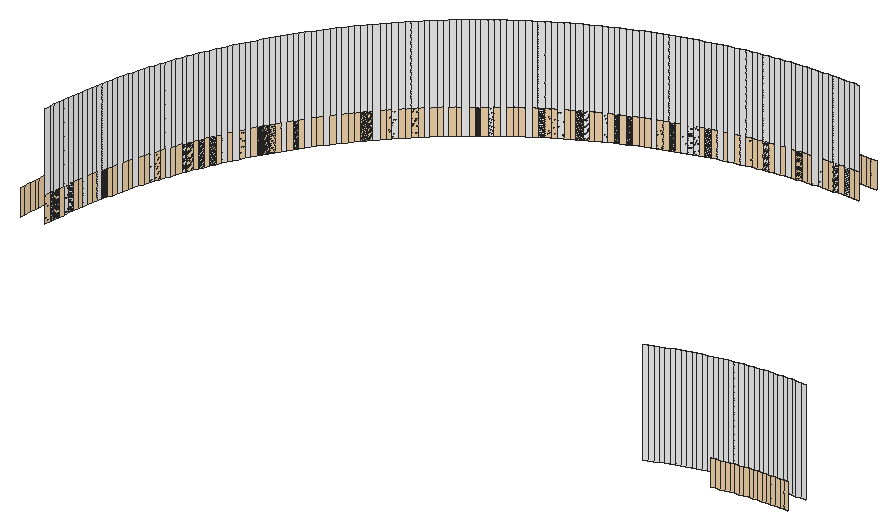
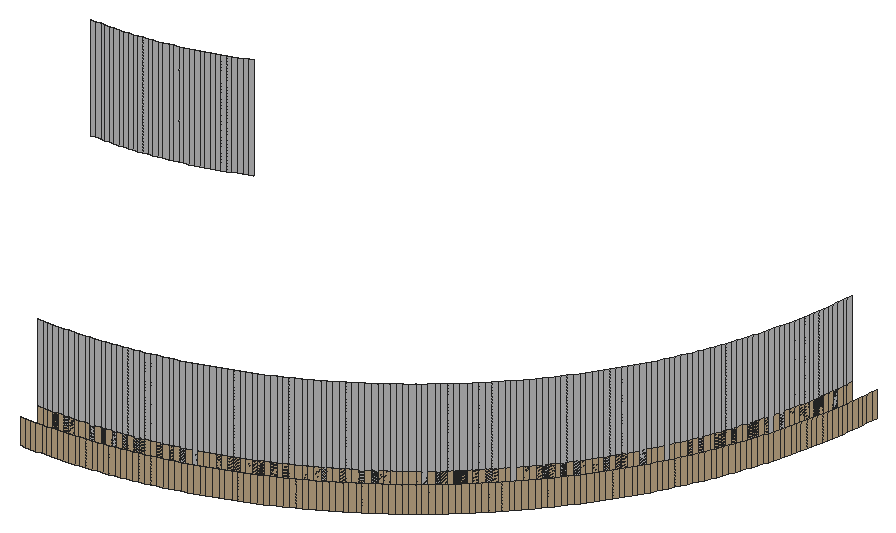
# SketchUp Ruby script. Lengths in inches.
U = 1.inch
M = Sketchup.active_model
def pt(a) = Geom::Point3d.new(a.map { |v| v * U })
def face(e, loops, mat)
  f = e.add_face(loops[0].map { |a| pt(a) })
  loops[1..].each { |l| e.add_face(l.map { |a| pt(a) }).erase! }
  f.material = f.back_material = mat if mat
  f
end
# faces: each face lists its corners as indices into pts; further lists are holes
def faces(e, pts, list, mat = nil) = list.each { |f| face(e, (f[0].is_a?(Array) ? f : [f]).map { |l| l.map { |i| pts[i] } }, mat) }
# xy, xz, yz: faces in a plane at the given z, y or x. An outline is a flat list of corners, or four numbers for a rectangle; further outlines are holes
def ring(l) = l.size == 4 ? [[l[0], l[1]], [l[2], l[1]], [l[2], l[3]], [l[0], l[3]]] : l.each_slice(2).to_a
def flat(e, list, mat, &to3) = list.each { |f| face(e, (f[0].is_a?(Array) ? f : [f]).map { |l| ring(l).map { |u, v| to3.(u, v) } }, mat) }
def xy(e, z, list, mat = nil) = flat(e, list, mat) { |x, y| [x, y, z] }
def xz(e, y, list, mat = nil) = flat(e, list, mat) { |x, z| [x, y, z] }
def yz(e, x, list, mat = nil) = flat(e, list, mat) { |y, z| [x, y, z] }
def lines(e, pts, list) = list.each { |a, b| e.add_line(pt(pts[a]), pt(pts[b])) }
# prism: a flat outline (further loops are holes) pulled along v
def prism(e, loops, v, mat = nil)
  f = face(e, loops, mat); d = Geom::Vector3d.new(v.map { |x| x * U })
  f.pushpull(f.normal.samedirection?(d) ? d.length : -d.length)
end
def box(e, o, s, mat = nil) = prism(e, [[o, [o[0] + s[0], o[1], o[2]], [o[0] + s[0], o[1] + s[1], o[2]], [o[0], o[1] + s[1], o[2]]]], [0, 0, s[2]], mat)
def at(x, y, z, deg = 0) = Geom::Transformation.translation(pt([x, y, z])) * Geom::Transformation.rotation(ORIGIN, Z_AXIS, deg.degrees)
def axes(o, x, y, z) = Geom::Transformation.new([*x, 0, *y, 0, *z, 0, *pt(o).to_a, 1])
def part(name) = M.definitions.add(name)
# library, detail: a bought-in or finely detailed component or shape, given as its bounding box
def library(name, o, s) = part(name).tap { |d| box(d.entities, o, s) }
def detail(e, o, s) = box(e.add_group.entities, o, s)
def put(e, d, t, mat = nil) = e.add_instance(d, t).tap { |i| i.material = mat if mat }
def group(e, t, mat = nil) = e.add_group.tap { |g| g.transformation = t; g.material = mat if mat }.entities
root = M.entities
M.materials.add("False Ceiling Light").color = [254, 223, 179]
M.materials.add("[Quartz Light Grey]").color = [251, 251, 252]
xz(root,218.5,[[56.62,115.32,56.81,116.49],[56.81,115.32,56.99,116.49]],"False Ceiling Light")
xz(root,219.49,[[56.39,115.32,56.59,120]],"[Quartz Light Grey]")
xz(root,219.5,[[56.8,115.32,56.99,120]],"[Quartz Light Grey]")
xz(root,237.5,[[44.55,115.32,44.77,116.49],[44.77,115.32,45.01,116.49]],"False Ceiling Light")
xz(root,237.5,[[44.55,115.32,44.77,120],[44.77,115.32,45.01,120]],"[Quartz Light Grey]")
xz(root,238.5,[[44.53,115.32,44.76,116.49],[44.76,115.32,45,116.49]],"False Ceiling Light")
p = [[22.625,218.35,115.32],[22.6,218.12,115.32],[22.6,218.12,116.49],[22.625,218.35,116.49],[53.99,218.18,115.32],[53.8,218.14,115.32],
  [53.8,218.14,116.49],[53.99,218.18,116.49],[23.64,218.47,115.32],[23.62,218.25,115.32],[23.62,218.25,120],[23.64,218.47,120],
  [23.62,218.25,115.32],[23.64,218.47,115.32],[23.64,218.47,116.49],[23.62,218.25,116.49],[50.7,218.16,115.32],[50.88,218.24,115.32],
  [50.88,218.24,120],[50.7,218.16,120],[51.07,218.32,115.32],[51.07,218.32,120],[54.17,218.22,115.32],[54.17,218.22,116.49],
  [54.36,218.26,115.32],[54.36,218.26,116.49],[51.26,218.4,115.32],[51.26,218.4,120],[54.54,218.29,115.32],[54.54,218.29,116.49],
  [54.73,218.32,115.32],[54.73,218.32,116.49],[54.92,218.35,115.32],[54.92,218.35,116.49],[55.11,218.375,115.32],[55.11,218.375,116.49],
  [22.65,218.59,115.32],[22.65,218.59,116.49],[51.45,218.47,115.32],[51.45,218.47,120],[55.3,218.4,115.32],[55.3,218.4,116.49],
  [55.48,218.42,115.32],[55.48,218.42,116.49],[55.67,218.4375,115.32],[55.67,218.4375,116.49],[55.86,218.46,115.32],[55.86,218.46,116.49],
  [23.67,218.69,115.32],[23.67,218.69,120],[23.67,218.69,115.32],[23.67,218.69,116.49],[51.64,218.54,115.32],[51.64,218.54,120],
  [51.83,218.61,115.32],[51.83,218.61,120],[56.05,218.47,115.32],[56.05,218.47,116.49],[56.24,218.48,115.32],[56.24,218.48,116.49],
  [56.43,218.49,115.32],[56.43,218.49,116.49],[56.62,218.5,115.32],[56.62,218.5,116.49],[22.68,218.82,115.32],[22.68,218.82,116.49],
  [52.02,218.68,115.32],[52.02,218.68,120],[23.7,218.92,115.32],[23.7,218.92,120],[23.7,218.92,115.32],[23.7,218.92,116.49],
  [52.21,218.74,115.32],[52.21,218.74,120],[52.4,218.8,115.32],[52.4,218.8,120],[22.71,219.05,115.32],[22.71,219.05,116.49],
  [52.6,218.86,115.32],[52.6,218.86,120],[23.73,219.14,115.32],[23.73,219.14,120],[23.73,219.14,115.32],[23.73,219.14,116.49],
  [52.79,218.92,115.32],[52.79,218.92,120],[52.99,218.97,115.32],[52.99,218.97,120],[53.18,219.02,115.32],[53.18,219.02,120],
  [53.38,219.07,115.32],[53.38,219.07,120],[22.74,219.29,115.32],[22.74,219.29,116.49],[23.76,219.36,115.32],[23.76,219.36,120],
  [23.76,219.36,115.32],[23.76,219.36,116.49],[53.58,219.12,115.32],[53.58,219.12,120],[53.78,219.16,115.32],[53.78,219.16,120],
  [53.98,219.2,115.32],[53.98,219.2,120],[54.18,219.24,115.32],[54.18,219.24,120],[54.375,219.28,115.32],[54.375,219.28,120],
  [22.78,219.52,115.32],[22.78,219.52,116.49],[54.58,219.31,115.32],[54.58,219.31,120],[54.78,219.34,115.32],[54.78,219.34,120],
  [54.98,219.37,115.32],[54.98,219.37,120],[23.8,219.59,115.32],[23.8,219.59,120],[23.8,219.59,115.32],[23.8,219.59,116.49],
  [55.18,219.39,115.32],[55.18,219.39,120],[55.38,219.42,115.32],[55.38,219.42,120],[55.58,219.44,115.32],[55.58,219.44,120],
  [55.78,219.45,115.32],[55.78,219.45,120],[22.82,219.75,115.32],[22.82,219.75,116.49],[55.99,219.47,115.32],[55.99,219.47,120],
  [56.1875,219.48,115.32],[56.1875,219.48,120],[56.39,219.49,115.32],[56.39,219.49,120],[56.59,219.49,115.32],[56.8,219.5,115.32],
  [56.8,219.5,120],[56.59,219.49,120],[23.84,219.81,115.32],[23.84,219.81,120],[23.84,219.81,115.32],[23.84,219.81,116.49],
  [22.86,219.98,115.32],[22.86,219.98,116.49],[23.88,220.03,115.32],[23.88,220.03,120],[23.88,220.03,115.32],[23.88,220.03,116.49],
  [22.9,220.22,115.32],[22.9,220.22,116.49],[23.92,220.25,115.32],[23.92,220.25,120],[23.92,220.25,115.32],[23.92,220.25,116.49],
  [22.94,220.45,115.32],[22.94,220.45,116.49],[23.97,220.47,115.32],[23.97,220.47,120],[23.97,220.47,115.32],[23.97,220.47,116.49],
  [22.99,220.68,115.32],[22.99,220.68,116.49],[24.02,220.69,115.32],[24.02,220.69,120],[24.02,220.69,115.32],[24.02,220.69,116.49],
  [23.04,220.91,115.32],[23.04,220.91,116.49],[24.07,220.91,115.32],[24.07,220.91,120],[24.07,220.91,115.32],[24.07,220.91,116.49],
  [23.09,221.14,115.32],[23.09,221.14,116.49],[24.12,221.13,115.32],[24.12,221.13,120],[24.12,221.13,115.32],[24.12,221.13,116.49],
  [23.15,221.37,115.32],[23.15,221.37,116.49],[24.18,221.35,115.32],[24.18,221.35,120],[24.18,221.35,115.32],[24.18,221.35,116.49],
  [24.23,221.56,115.32],[24.23,221.56,120],[24.23,221.56,115.32],[24.23,221.56,116.49],[23.21,221.6,115.32],[23.21,221.6,116.49],
  [23.27,221.82,115.32],[23.27,221.82,116.49],[24.29,221.78,115.32],[24.29,221.78,120],[24.29,221.78,115.32],[24.29,221.78,116.49],
  [23.33,222.05,115.32],[23.33,222.05,116.49],[24.35,222,115.32],[24.35,222,120],[24.35,222,115.32],[24.35,222,116.49],
  [24.42,222.21,115.32],[24.42,222.21,120],[24.42,222.21,115.32],[24.42,222.21,116.49],[23.39,222.28,115.32],[23.39,222.28,116.49],
  [24.48,222.43,115.32],[24.48,222.43,120],[24.48,222.43,115.32],[24.48,222.43,116.49],[23.46,222.5,115.32],[23.46,222.5,116.49],
  [24.55,222.64,115.32],[24.55,222.64,120],[24.55,222.64,115.32],[24.55,222.64,116.49],[23.53,222.73,115.32],[23.53,222.73,116.49],
  [24.625,222.86,115.32],[24.625,222.86,120],[24.625,222.86,115.32],[24.625,222.86,116.49],[23.6,222.95,115.32],[23.6,222.95,116.49],
  [24.7,223.07,115.32],[24.7,223.07,120],[24.7,223.07,115.32],[24.7,223.07,116.49],[23.68,223.18,115.32],[23.68,223.18,116.49],
  [24.77,223.28,115.32],[24.77,223.28,120],[24.77,223.28,115.32],[24.77,223.28,116.49],[23.75,223.4,115.32],[23.75,223.4,116.49],
  [24.85,223.49,115.32],[24.85,223.49,120],[24.85,223.49,115.32],[24.85,223.49,116.49],[23.83,223.62,115.32],[23.83,223.62,116.49],
  [24.93,223.7,115.32],[24.93,223.7,120],[24.93,223.7,115.32],[24.93,223.7,116.49],[23.91,223.84,115.32],[23.91,223.84,116.49],
  [25.01,223.91,115.32],[25.01,223.91,120],[25.01,223.91,115.32],[25.01,223.91,116.49],[23.99,224.0625,115.32],[23.99,224.0625,116.49],
  [25.09,224.125,115.32],[25.09,224.125,120],[25.09,224.125,115.32],[25.09,224.125,116.49],[24.08,224.28,115.32],[24.08,224.28,116.49],
  [25.18,224.33,115.32],[25.18,224.33,120],[25.18,224.33,115.32],[25.18,224.33,116.49],[24.17,224.5,115.32],[24.17,224.5,116.49],
  [25.27,224.54,115.32],[25.27,224.54,120],[25.27,224.54,115.32],[25.27,224.54,116.49],[24.26,224.72,115.32],[24.26,224.72,116.49],
  [25.36,224.74,115.32],[25.36,224.74,120],[25.36,224.74,115.32],[25.36,224.74,116.49],[24.35,224.9375,115.32],[24.35,224.9375,116.49],
  [25.45,224.95,115.32],[25.45,224.95,120],[25.45,224.95,115.32],[25.45,224.95,116.49],[24.45,225.15,115.32],[24.45,225.15,116.49],
  [25.55,225.15,115.32],[25.55,225.15,120],[25.55,225.15,115.32],[25.55,225.15,116.49],[24.54,225.37,115.32],[24.54,225.37,116.49],
  [25.64,225.36,115.32],[25.64,225.36,120],[25.64,225.36,115.32],[25.64,225.36,116.49],[24.64,225.58,115.32],[24.64,225.58,116.49],
  [25.74,225.56,115.32],[25.74,225.56,120],[25.74,225.56,115.32],[25.74,225.56,116.49],[24.74,225.79,115.32],[24.74,225.79,116.49],
  [25.84,225.76,115.32],[25.84,225.76,120],[25.84,225.76,115.32],[25.84,225.76,116.49],[24.85,226,115.32],[24.85,226,116.49],
  [25.95,225.96,115.32],[25.95,225.96,120],[25.95,225.96,115.32],[25.95,225.96,116.49],[24.95,226.21,115.32],[24.95,226.21,116.49],
  [26.05,226.16,115.32],[26.05,226.16,120],[26.05,226.16,115.32],[26.05,226.16,116.49],[25.06,226.42,115.32],[25.06,226.42,116.49],
  [26.16,226.36,115.32],[26.16,226.36,120],[26.16,226.36,115.32],[26.16,226.36,116.49],[25.17,226.63,115.32],[25.17,226.63,116.49],
  [26.27,226.55,115.32],[26.27,226.55,120],[26.27,226.55,115.32],[26.27,226.55,116.49],[25.28,226.84,115.32],[25.28,226.84,116.49],
  [26.38,226.75,115.32],[26.38,226.75,120],[26.38,226.75,115.32],[26.38,226.75,116.49],[26.49,226.94,115.32],[26.49,226.94,120],
  [26.49,226.94,115.32],[26.49,226.94,116.49],[25.4,227.05,115.32],[25.4,227.05,116.49],[26.61,227.14,115.32],[26.61,227.14,120],
  [26.61,227.14,115.32],[26.61,227.14,116.49],[25.51,227.25,115.32],[25.51,227.25,116.49],[26.73,227.33,115.32],[26.73,227.33,120],
  [26.73,227.33,115.32],[26.73,227.33,116.49],[25.63,227.45,115.32],[25.63,227.45,116.49],[26.85,227.52,115.32],[26.85,227.52,120],
  [26.85,227.52,115.32],[26.85,227.52,116.49],[25.75,227.66,115.32],[25.75,227.66,116.49],[26.97,227.71,115.32],[26.97,227.71,120],
  [26.97,227.71,115.32],[26.97,227.71,116.49],[25.88,227.86,115.32],[25.88,227.86,116.49],[27.09,227.9,115.32],[27.09,227.9,120],
  [27.09,227.9,115.32],[27.09,227.9,116.49],[26,228.06,115.32],[26,228.06,116.49],[27.22,228.08,115.32],[27.22,228.08,120],
  [27.22,228.08,115.32],[27.22,228.08,116.49],[26.13,228.25,115.32],[26.13,228.25,116.49],[27.35,228.27,115.32],[27.35,228.27,120],
  [27.35,228.27,115.32],[27.35,228.27,116.49],[26.26,228.45,115.32],[26.26,228.45,116.49],[27.47,228.45,115.32],[27.47,228.45,120],
  [27.47,228.45,115.32],[27.47,228.45,116.49],[26.39,228.65,115.32],[26.39,228.65,116.49],[27.61,228.64,115.32],[27.61,228.64,120],
  [27.61,228.64,115.32],[27.61,228.64,116.49],[26.52,228.84,115.32],[26.52,228.84,116.49],[27.74,228.82,115.32],[27.74,228.82,120],
  [27.74,228.82,115.32],[27.74,228.82,116.49],[26.66,229.03,115.32],[26.66,229.03,116.49],[27.875,229,115.32],[27.875,229,120],
  [27.875,229,115.32],[27.875,229,116.49],[26.8,229.23,115.32],[26.8,229.23,116.49],[28.01,229.18,115.32],[28.01,229.18,120],
  [28.01,229.18,115.32],[28.01,229.18,116.49],[26.9375,229.42,115.32],[26.9375,229.42,116.49],[28.15,229.35,115.32],[28.15,229.35,120],
  [28.15,229.35,115.32],[28.15,229.35,116.49],[27.08,229.6,115.32],[27.08,229.6,116.49],[28.29,229.53,115.32],[28.29,229.53,120],
  [28.29,229.53,115.32],[28.29,229.53,116.49],[28.43,229.7,115.32],[28.43,229.7,120],[28.43,229.7,115.32],[28.43,229.7,116.49],
  [27.22,229.79,115.32],[27.22,229.79,116.49],[28.58,229.88,115.32],[28.58,229.88,120],[28.58,229.88,115.32],[28.58,229.88,116.49],
  [27.37,229.98,115.32],[27.37,229.98,116.49],[28.72,230.05,115.32],[28.72,230.05,120],[28.72,230.05,115.32],[28.72,230.05,116.49],
  [27.51,230.16,115.32],[27.51,230.16,116.49],[28.87,230.22,115.32],[28.87,230.22,120],[28.87,230.22,115.32],[28.87,230.22,116.49],
  [27.66,230.34,115.32],[27.66,230.34,116.49],[29.02,230.39,115.32],[29.02,230.39,120],[29.02,230.39,115.32],[29.02,230.39,116.49],
  [27.81,230.52,115.32],[27.81,230.52,116.49],[29.17,230.55,115.32],[29.17,230.55,120],[29.17,230.55,115.32],[29.17,230.55,116.49],
  [27.97,230.7,115.32],[27.97,230.7,116.49],[29.33,230.72,115.32],[29.33,230.72,120],[29.33,230.72,115.32],[29.33,230.72,116.49],
  [28.12,230.88,115.32],[28.12,230.88,116.49],[29.48,230.88,115.32],[29.48,230.88,120],[29.48,230.88,115.32],[29.48,230.88,116.49],
  [28.28,231.06,115.32],[28.28,231.06,116.49],[29.64,231.04,115.32],[29.64,231.04,120],[29.64,231.04,115.32],[29.64,231.04,116.49],
  [29.8,231.2,115.32],[29.8,231.2,120],[29.8,231.2,115.32],[29.8,231.2,116.49],[28.4375,231.23,115.32],[28.4375,231.23,116.49],
  [28.6,231.4,115.32],[28.6,231.4,116.49],[29.96,231.36,115.32],[29.96,231.36,120],[29.96,231.36,115.32],[29.96,231.36,116.49],
  [28.76,231.57,115.32],[28.76,231.57,116.49],[30.12,231.52,115.32],[30.12,231.52,120],[30.12,231.52,115.32],[30.12,231.52,116.49],
  [30.28,231.67,115.32],[30.28,231.67,120],[30.28,231.67,115.32],[30.28,231.67,116.49],[28.92,231.74,115.32],[28.92,231.74,116.49],
  [29.09,231.91,115.32],[29.09,231.91,116.49],[30.45,231.83,115.32],[30.45,231.83,120],[30.45,231.83,115.32],[30.45,231.83,116.49],
  [30.61,231.98,115.32],[30.61,231.98,120],[30.61,231.98,115.32],[30.61,231.98,116.49],[29.26,232.08,115.32],[29.26,232.08,116.49],
  [30.78,232.13,115.32],[30.78,232.13,120],[30.78,232.13,115.32],[30.78,232.13,116.49],[29.43,232.24,115.32],[29.43,232.24,116.49],
  [30.95,232.28,115.32],[30.95,232.28,120],[30.95,232.28,115.32],[30.95,232.28,116.49],[29.6,232.4,115.32],[29.6,232.4,116.49],
  [31.12,232.42,115.32],[31.12,232.42,120],[31.12,232.42,115.32],[31.12,232.42,116.49],[29.77,232.5625,115.32],[29.77,232.5625,116.49],
  [31.3,232.57,115.32],[31.3,232.57,120],[31.3,232.57,115.32],[31.3,232.57,116.49],[29.94,232.72,115.32],[29.94,232.72,116.49],
  [31.47,232.71,115.32],[31.47,232.71,120],[31.47,232.71,115.32],[31.47,232.71,116.49],[30.12,232.88,115.32],[30.12,232.88,116.49],
  [31.65,232.85,115.32],[31.65,232.85,120],[31.65,232.85,115.32],[31.65,232.85,116.49],[31.82,232.99,115.32],[31.82,232.99,120],
  [31.82,232.99,115.32],[31.82,232.99,116.49],[30.3,233.03,115.32],[30.3,233.03,116.49],[30.48,233.19,115.32],[30.48,233.19,116.49],
  [32,233.125,115.32],[32,233.125,120],[32,233.125,115.32],[32,233.125,116.49],[32.18,233.26,115.32],[32.18,233.26,120],
  [32.18,233.26,115.32],[32.18,233.26,116.49],[30.66,233.34,115.32],[30.66,233.34,116.49],[30.84,233.49,115.32],[30.84,233.49,116.49],
  [32.36,233.39,115.32],[32.36,233.39,120],[32.36,233.39,115.32],[32.36,233.39,116.49],[32.55,233.53,115.32],[32.55,233.53,120],
  [32.55,233.53,115.32],[32.55,233.53,116.49],[31.02,233.63,115.32],[31.02,233.63,116.49],[32.73,233.65,115.32],[32.73,233.65,120],
  [32.73,233.65,115.32],[32.73,233.65,116.49],[31.21,233.78,115.32],[31.21,233.78,116.49],[32.92,233.78,115.32],[32.92,233.78,120],
  [32.92,233.78,115.32],[32.92,233.78,116.49],[31.4,233.92,115.32],[31.4,233.92,116.49],[33.1,233.91,115.32],[33.1,233.91,120],
  [33.1,233.91,115.32],[33.1,233.91,116.49],[31.58,234.0625,115.32],[31.58,234.0625,116.49],[33.29,234.03,115.32],[33.29,234.03,120],
  [33.29,234.03,115.32],[33.29,234.03,116.49],[33.48,234.15,115.32],[33.48,234.15,120],[33.48,234.15,115.32],[33.48,234.15,116.49],
  [31.77,234.2,115.32],[31.77,234.2,116.49],[31.97,234.34,115.32],[31.97,234.34,116.49],[33.67,234.27,115.32],[33.67,234.27,120],
  [33.67,234.27,115.32],[33.67,234.27,116.49],[32.16,234.48,115.32],[32.16,234.48,116.49],[33.86,234.39,115.32],[33.86,234.39,120],
  [33.86,234.39,115.32],[33.86,234.39,116.49],[34.06,234.51,115.32],[34.06,234.51,120],[34.06,234.51,115.32],[34.06,234.51,116.49],
  [32.35,234.61,115.32],[32.35,234.61,116.49],[34.25,234.62,115.32],[34.25,234.62,120],[34.25,234.62,115.32],[34.25,234.62,116.49],
  [32.55,234.74,115.32],[32.55,234.74,116.49],[34.45,234.73,115.32],[34.45,234.73,120],[34.45,234.73,115.32],[34.45,234.73,116.49],
  [32.75,234.87,115.32],[32.75,234.87,116.49],[34.64,234.84,115.32],[34.64,234.84,120],[34.64,234.84,115.32],[34.64,234.84,116.49],
  [34.84,234.95,115.32],[34.84,234.95,120],[34.84,234.95,115.32],[34.84,234.95,116.49],[32.94,235,115.32],[32.94,235,116.49],
  [35.04,235.05,115.32],[35.04,235.05,120],[35.04,235.05,115.32],[35.04,235.05,116.49],[33.14,235.12,115.32],[33.14,235.12,116.49],
  [33.34,235.25,115.32],[33.34,235.25,116.49],[35.24,235.16,115.32],[35.24,235.16,120],[35.24,235.16,115.32],[35.24,235.16,116.49],
  [33.55,235.37,115.32],[33.55,235.37,116.49],[35.44,235.26,115.32],[35.44,235.26,120],[35.44,235.26,115.32],[35.44,235.26,116.49],
  [35.64,235.36,115.32],[35.64,235.36,120],[35.64,235.36,115.32],[35.64,235.36,116.49],[33.75,235.49,115.32],[33.75,235.49,116.49],
  [35.85,235.45,115.32],[35.85,235.45,120],[35.85,235.45,115.32],[35.85,235.45,116.49],[33.95,235.6,115.32],[33.95,235.6,116.49],
  [36.05,235.55,115.32],[36.05,235.55,120],[36.05,235.55,115.32],[36.05,235.55,116.49],[36.26,235.64,115.32],[36.26,235.64,120],
  [36.26,235.64,115.32],[36.26,235.64,116.49],[34.16,235.72,115.32],[34.16,235.72,116.49],[36.46,235.73,115.32],[36.46,235.73,120],
  [36.46,235.73,115.32],[36.46,235.73,116.49],[34.37,235.83,115.32],[34.37,235.83,116.49],[36.67,235.82,115.32],[36.67,235.82,120],
  [36.67,235.82,115.32],[36.67,235.82,116.49],[34.58,235.94,115.32],[34.58,235.94,116.49],[36.875,235.91,115.32],[36.875,235.91,120],
  [36.875,235.91,115.32],[36.875,235.91,116.49],[34.79,236.05,115.32],[34.79,236.05,116.49],[37.09,235.99,115.32],[37.09,235.99,120],
  [37.09,235.99,115.32],[37.09,235.99,116.49],[35,236.15,115.32],[35,236.15,116.49],[37.3,236.07,115.32],[37.3,236.07,120],
  [37.3,236.07,115.32],[37.3,236.07,116.49],[37.51,236.15,115.32],[37.51,236.15,120],[37.51,236.15,115.32],[37.51,236.15,116.49],
  [35.21,236.26,115.32],[35.21,236.26,116.49],[37.72,236.23,115.32],[37.72,236.23,120],[37.72,236.23,115.32],[37.72,236.23,116.49],
  [37.93,236.3,115.32],[37.93,236.3,120],[37.93,236.3,115.32],[37.93,236.3,116.49],[35.42,236.36,115.32],[35.42,236.36,116.49],
  [38.14,236.375,115.32],[38.14,236.375,120],[38.14,236.375,115.32],[38.14,236.375,116.49],[35.63,236.46,115.32],[35.63,236.46,116.49],
  [38.36,236.45,115.32],[38.36,236.45,120],[38.36,236.45,115.32],[38.36,236.45,116.49],[38.57,236.52,115.32],[38.57,236.52,120],
  [38.57,236.52,115.32],[38.57,236.52,116.49],[35.85,236.55,115.32],[35.85,236.55,116.49],[38.79,236.58,115.32],[38.79,236.58,120],
  [38.79,236.58,115.32],[38.79,236.58,116.49],[36.0625,236.65,115.32],[36.0625,236.65,116.49],[36.28,236.74,115.32],[36.28,236.74,116.49],
  [39,236.65,115.32],[39,236.65,120],[39,236.65,115.32],[39,236.65,116.49],[39.22,236.71,115.32],[39.22,236.71,120],
  [39.22,236.71,115.32],[39.22,236.71,116.49],[36.5,236.83,115.32],[36.5,236.83,116.49],[39.44,236.77,115.32],[39.44,236.77,120],
  [39.44,236.77,115.32],[39.44,236.77,116.49],[36.72,236.92,115.32],[36.72,236.92,116.49],[39.65,236.82,115.32],[39.65,236.82,120],
  [39.65,236.82,115.32],[39.65,236.82,116.49],[39.87,236.88,115.32],[39.87,236.88,120],[39.87,236.88,115.32],[39.87,236.88,116.49],
  [36.9375,237.01,115.32],[36.9375,237.01,116.49],[40.09,236.93,115.32],[40.09,236.93,120],[40.09,236.93,115.32],[40.09,236.93,116.49],
  [40.31,236.98,115.32],[40.31,236.98,120],[40.31,236.98,115.32],[40.31,236.98,116.49],[37.16,237.09,115.32],[37.16,237.09,116.49],
  [40.53,237.03,115.32],[40.53,237.03,120],[40.53,237.03,115.32],[40.53,237.03,116.49],[40.75,237.08,115.32],[40.75,237.08,120],
  [40.75,237.08,115.32],[40.75,237.08,116.49],[37.38,237.17,115.32],[37.38,237.17,116.49],[40.97,237.12,115.32],[40.97,237.12,120],
  [40.97,237.12,115.32],[40.97,237.12,116.49],[41.19,237.16,115.32],[41.19,237.16,120],[41.19,237.16,115.32],[41.19,237.16,116.49],
  [37.6,237.25,115.32],[37.6,237.25,116.49],[37.82,237.32,115.32],[37.82,237.32,116.49],[41.41,237.2,115.32],[41.41,237.2,120],
  [41.41,237.2,115.32],[41.41,237.2,116.49],[41.64,237.24,115.32],[41.64,237.24,120],[41.64,237.24,115.32],[41.64,237.24,116.49],
  [41.86,237.27,115.32],[41.86,237.27,120],[41.86,237.27,115.32],[41.86,237.27,116.49],[38.05,237.4,115.32],[38.05,237.4,116.49],
  [42.08,237.3,115.32],[42.08,237.3,120],[42.08,237.3,115.32],[42.08,237.3,116.49],[42.31,237.33,115.32],[42.31,237.33,120],
  [42.31,237.33,115.32],[42.31,237.33,116.49],[42.53,237.36,115.32],[42.53,237.36,120],[42.53,237.36,115.32],[42.53,237.36,116.49],
  [38.27,237.47,115.32],[38.27,237.47,116.49],[42.75,237.38,115.32],[42.75,237.38,120],[42.75,237.38,115.32],[42.75,237.38,116.49],
  [42.98,237.4,115.32],[42.98,237.4,120],[42.98,237.4,115.32],[42.98,237.4,116.49],[43.2,237.42,115.32],[43.2,237.42,120],
  [43.2,237.42,115.32],[43.2,237.42,116.49],[43.43,237.44,115.32],[43.43,237.44,120],[43.43,237.44,115.32],[43.43,237.44,116.49],
  [43.65,237.46,115.32],[43.65,237.46,120],[43.65,237.46,115.32],[43.65,237.46,116.49],[38.5,237.54,115.32],[38.5,237.54,116.49],
  [38.72,237.61,115.32],[38.72,237.61,116.49],[43.875,237.47,115.32],[43.875,237.47,120],[43.875,237.47,115.32],[43.875,237.47,116.49],
  [44.1,237.48,115.32],[44.1,237.48,120],[44.1,237.48,115.32],[44.1,237.48,116.49],[44.32,237.49,115.32],[44.32,237.49,120],
  [44.32,237.49,115.32],[44.32,237.49,116.49],[44.55,237.5,115.32],[44.55,237.5,120],[44.55,237.5,115.32],[44.55,237.5,116.49],
  [38.95,237.67,115.32],[38.95,237.67,116.49],[39.18,237.73,115.32],[39.18,237.73,116.49],[39.4,237.79,115.32],[39.4,237.79,116.49],
  [39.63,237.85,115.32],[39.63,237.85,116.49],[39.86,237.91,115.32],[39.86,237.91,116.49],[40.09,237.96,115.32],[40.09,237.96,116.49],
  [40.32,238.01,115.32],[40.32,238.01,116.49],[40.55,238.06,115.32],[40.55,238.06,116.49],[40.78,238.1,115.32],[40.78,238.1,116.49],
  [41.02,238.14,115.32],[41.02,238.14,116.49],[41.25,238.18,115.32],[41.25,238.18,116.49],[41.48,238.22,115.32],[41.48,238.22,116.49],
  [41.71,238.26,115.32],[41.71,238.26,116.49],[41.95,238.29,115.32],[41.95,238.29,116.49],[42.18,238.32,115.32],[42.18,238.32,116.49],
  [42.41,238.35,115.32],[42.41,238.35,116.49],[42.65,238.375,115.32],[42.65,238.375,116.49],[42.88,238.4,115.32],[42.88,238.4,116.49],
  [43.12,238.42,115.32],[43.12,238.42,116.49],[43.35,238.44,115.32],[43.35,238.44,116.49],[43.59,238.46,115.32],[43.59,238.46,116.49],
  [43.82,238.47,115.32],[43.82,238.47,116.49],[44.06,238.48,115.32],[44.06,238.48,116.49],[44.29,238.49,115.32],[44.29,238.49,116.49],
  [44.53,238.5,115.32],[44.53,238.5,116.49]]
faces(root,p,[[0,1,2,3],[4,5,6,7],[12,13,14,15],[22,4,7,23],[24,22,23,25],[28,24,25,29],[30,28,29,31],[32,30,31,33],
  [34,32,33,35],[36,0,3,37],[40,34,35,41],[42,40,41,43],[44,42,43,45],[46,44,45,47],[13,50,51,14],[56,46,47,57],
  [58,56,57,59],[60,58,59,61],[62,60,61,63],[64,36,37,65],[50,70,71,51],[76,64,65,77],[70,82,83,71],[92,76,77,93],
  [82,96,97,83],[108,92,93,109],[96,118,119,97],[128,108,109,129],[118,142,143,119],[144,128,129,145],[142,148,149,143],[150,144,145,151],
  [148,154,155,149],[156,150,151,157],[154,160,161,155],[162,156,157,163],[160,166,167,161],[168,162,163,169],[166,172,173,167],[174,168,169,175],
  [172,178,179,173],[180,174,175,181],[178,184,185,179],[184,188,189,185],[190,180,181,191],[192,190,191,193],[188,196,197,189],[198,192,193,199],
  [196,202,203,197],[202,206,207,203],[208,198,199,209],[206,212,213,207],[214,208,209,215],[212,218,219,213],[220,214,215,221],[218,224,225,219],
  [226,220,221,227],[224,230,231,225],[232,226,227,233],[230,236,237,231],[238,232,233,239],[236,242,243,237],[244,238,239,245],[242,248,249,243],
  [250,244,245,251],[248,254,255,249],[256,250,251,257],[254,260,261,255],[262,256,257,263],[260,266,267,261],[268,262,263,269],[266,272,273,267],
  [274,268,269,275],[272,278,279,273],[280,274,275,281],[278,284,285,279],[286,280,281,287],[284,290,291,285],[292,286,287,293],[290,296,297,291],
  [298,292,293,299],[296,302,303,297],[304,298,299,305],[302,308,309,303],[310,304,305,311],[308,314,315,309],[316,310,311,317],[314,320,321,315],
  [322,316,317,323],[320,326,327,321],[328,322,323,329],[326,332,333,327],[334,328,329,335],[332,338,339,333],[338,342,343,339],[344,334,335,345],
  [342,348,349,343],[350,344,345,351],[348,354,355,349],[356,350,351,357],[354,360,361,355],[362,356,357,363],[360,366,367,361],[368,362,363,369],
  [366,372,373,367],[374,368,369,375],[372,378,379,373],[380,374,375,381],[378,384,385,379],[386,380,381,387],[384,390,391,385],[392,386,387,393],
  [390,396,397,391],[398,392,393,399],[396,402,403,397],[404,398,399,405],[402,408,409,403],[410,404,405,411],[408,414,415,409],[416,410,411,417],
  [414,420,421,415],[422,416,417,423],[420,426,427,421],[426,430,431,427],[432,422,423,433],[430,436,437,431],[438,432,433,439],[436,442,443,437],
  [444,438,439,445],[442,448,449,443],[450,444,445,451],[448,454,455,449],[456,450,451,457],[454,460,461,455],[462,456,457,463],[460,466,467,461],
  [468,462,463,469],[466,472,473,467],[474,468,469,475],[472,478,479,473],[478,482,483,479],[484,474,475,485],[486,484,485,487],[482,490,491,483],
  [492,486,487,493],[490,496,497,491],[496,500,501,497],[502,492,493,503],[504,502,503,505],[500,508,509,501],[508,512,513,509],[514,504,505,515],
  [512,518,519,513],[520,514,515,521],[518,524,525,519],[526,520,521,527],[524,530,531,525],[532,526,527,533],[530,536,537,531],[538,532,533,539],
  [536,542,543,537],[544,538,539,545],[542,548,549,543],[548,552,553,549],[554,544,545,555],[556,554,555,557],[552,560,561,553],[560,564,565,561],
  [566,556,557,567],[568,566,567,569],[564,572,573,565],[572,576,577,573],[578,568,569,579],[576,582,583,577],[584,578,579,585],[582,588,589,583],
  [590,584,585,591],[588,594,595,589],[596,590,591,597],[594,600,601,595],[600,604,605,601],[606,596,597,607],[608,606,607,609],[604,612,613,605],
  [614,608,609,615],[612,618,619,613],[618,622,623,619],[624,614,615,625],[622,628,629,623],[630,624,625,631],[628,634,635,629],[636,630,631,637],
  [634,640,641,635],[640,644,645,641],[646,636,637,647],[644,650,651,645],[652,646,647,653],[654,652,653,655],[650,658,659,651],[660,654,655,661],
  [658,664,665,659],[664,668,669,665],[670,660,661,671],[668,674,675,669],[676,670,671,677],[674,680,681,675],[680,684,685,681],[686,676,677,687],
  [684,690,691,685],[692,686,687,693],[690,696,697,691],[698,692,693,699],[696,702,703,697],[704,698,699,705],[702,708,709,703],[710,704,705,711],
  [708,714,715,709],[714,718,719,715],[720,710,711,721],[718,724,725,719],[724,728,729,725],[730,720,721,731],[728,734,735,729],[736,730,731,737],
  [734,740,741,735],[740,744,745,741],[746,736,737,747],[744,750,751,745],[752,746,747,753],[754,752,753,755],[750,758,759,751],[758,762,763,759],
  [764,754,755,765],[762,768,769,763],[770,764,765,771],[768,774,775,769],[774,778,779,775],[780,770,771,781],[778,784,785,779],[784,788,789,785],
  [790,780,781,791],[788,794,795,789],[794,798,799,795],[800,790,791,801],[798,804,805,799],[804,808,809,805],[810,800,801,811],[812,810,811,813],
  [808,816,817,809],[816,820,821,817],[820,824,825,821],[826,812,813,827],[824,830,831,825],[830,834,835,831],[834,838,839,835],[840,826,827,841],
  [838,844,845,839],[844,848,849,845],[848,852,853,849],[852,856,857,853],[856,860,861,857],[862,840,841,863],[864,862,863,865],[860,868,869,861],
  [868,872,873,869],[872,876,877,873],[876,880,881,877],[882,864,865,883],[884,882,883,885],[886,884,885,887],[888,886,887,889],[890,888,889,891],
  [892,890,891,893],[894,892,893,895],[896,894,895,897],[898,896,897,899],[900,898,899,901],[902,900,901,903],[904,902,903,905],[906,904,905,907],
  [908,906,907,909],[910,908,909,911],[912,910,911,913],[914,912,913,915],[916,914,915,917],[918,916,917,919],[920,918,919,921],[922,920,921,923],
  [924,922,923,925],[926,924,925,927],[928,926,927,929],[930,928,929,931]],"False Ceiling Light")
faces(root,p,[[8,9,10,11],[16,17,18,19],[17,20,21,18],[20,26,27,21],[26,38,39,27],[48,8,11,49],[38,52,53,39],[52,54,55,53],
  [54,66,67,55],[68,48,49,69],[66,72,73,67],[72,74,75,73],[74,78,79,75],[80,68,69,81],[78,84,85,79],[84,86,87,85],
  [86,88,89,87],[88,90,91,89],[94,80,81,95],[90,98,99,91],[98,100,101,99],[100,102,103,101],[102,104,105,103],[104,106,107,105],
  [106,110,111,107],[110,112,113,111],[112,114,115,113],[116,94,95,117],[114,120,121,115],[120,122,123,121],[122,124,125,123],[124,126,127,125],
  [126,130,131,127],[130,132,133,131],[132,134,135,133],[136,137,138,139],[140,116,117,141],[146,140,141,147],[152,146,147,153],[158,152,153,159],
  [164,158,159,165],[170,164,165,171],[176,170,171,177],[182,176,177,183],[186,182,183,187],[194,186,187,195],[200,194,195,201],[204,200,201,205],
  [210,204,205,211],[216,210,211,217],[222,216,217,223],[228,222,223,229],[234,228,229,235],[240,234,235,241],[246,240,241,247],[252,246,247,253],
  [258,252,253,259],[264,258,259,265],[270,264,265,271],[276,270,271,277],[282,276,277,283],[288,282,283,289],[294,288,289,295],[300,294,295,301],
  [306,300,301,307],[312,306,307,313],[318,312,313,319],[324,318,319,325],[330,324,325,331],[336,330,331,337],[340,336,337,341],[346,340,341,347],
  [352,346,347,353],[358,352,353,359],[364,358,359,365],[370,364,365,371],[376,370,371,377],[382,376,377,383],[388,382,383,389],[394,388,389,395],
  [400,394,395,401],[406,400,401,407],[412,406,407,413],[418,412,413,419],[424,418,419,425],[428,424,425,429],[434,428,429,435],[440,434,435,441],
  [446,440,441,447],[452,446,447,453],[458,452,453,459],[464,458,459,465],[470,464,465,471],[476,470,471,477],[480,476,477,481],[488,480,481,489],
  [494,488,489,495],[498,494,495,499],[506,498,499,507],[510,506,507,511],[516,510,511,517],[522,516,517,523],[528,522,523,529],[534,528,529,535],
  [540,534,535,541],[546,540,541,547],[550,546,547,551],[558,550,551,559],[562,558,559,563],[570,562,563,571],[574,570,571,575],[580,574,575,581],
  [586,580,581,587],[592,586,587,593],[598,592,593,599],[602,598,599,603],[610,602,603,611],[616,610,611,617],[620,616,617,621],[626,620,621,627],
  [632,626,627,633],[638,632,633,639],[642,638,639,643],[648,642,643,649],[656,648,649,657],[662,656,657,663],[666,662,663,667],[672,666,667,673],
  [678,672,673,679],[682,678,679,683],[688,682,683,689],[694,688,689,695],[700,694,695,701],[706,700,701,707],[712,706,707,713],[716,712,713,717],
  [722,716,717,723],[726,722,723,727],[732,726,727,733],[738,732,733,739],[742,738,739,743],[748,742,743,749],[756,748,749,757],[760,756,757,761],
  [766,760,761,767],[772,766,767,773],[776,772,773,777],[782,776,777,783],[786,782,783,787],[792,786,787,793],[796,792,793,797],[802,796,797,803],
  [806,802,803,807],[814,806,807,815],[818,814,815,819],[822,818,819,823],[828,822,823,829],[832,828,829,833],[836,832,833,837],[842,836,837,843],
  [846,842,843,847],[850,846,847,851],[854,850,851,855],[858,854,855,859],[866,858,859,867],[870,866,867,871],[874,870,871,875],[878,874,875,879]],"[Quartz Light Grey]")
